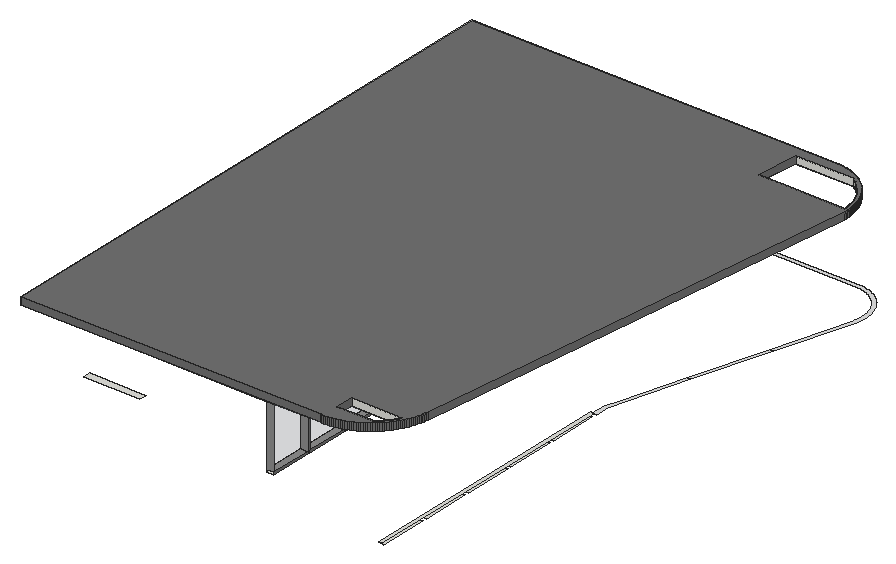
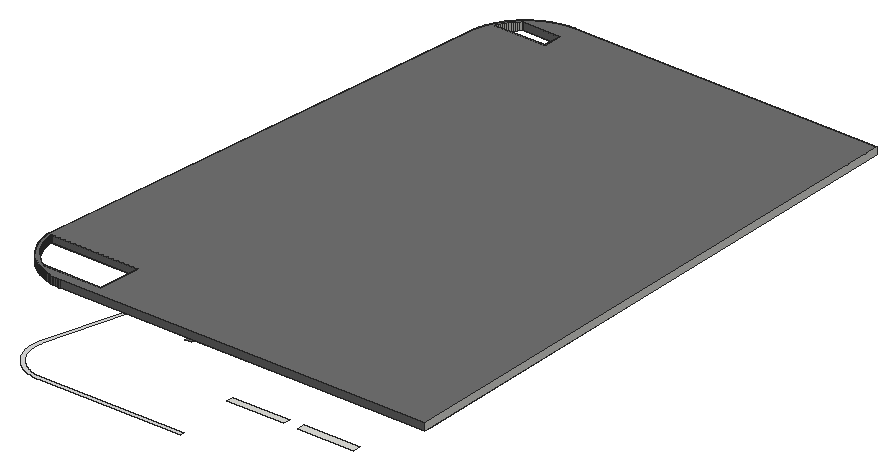
# SketchUp Ruby script. Lengths in inches.
U = 1.inch
M = Sketchup.active_model
def pt(a) = Geom::Point3d.new(a.map { |v| v * U })
def face(e, loops, mat)
  f = e.add_face(loops[0].map { |a| pt(a) })
  loops[1..].each { |l| e.add_face(l.map { |a| pt(a) }).erase! }
  f.material = f.back_material = mat if mat
  f
end
# faces: each face lists its corners as indices into pts; further lists are holes
def faces(e, pts, list, mat = nil) = list.each { |f| face(e, (f[0].is_a?(Array) ? f : [f]).map { |l| l.map { |i| pts[i] } }, mat) }
# xy, xz, yz: faces in a plane at the given z, y or x. An outline is a flat list of corners, or four numbers for a rectangle; further outlines are holes
def ring(l) = l.size == 4 ? [[l[0], l[1]], [l[2], l[1]], [l[2], l[3]], [l[0], l[3]]] : l.each_slice(2).to_a
def flat(e, list, mat, &to3) = list.each { |f| face(e, (f[0].is_a?(Array) ? f : [f]).map { |l| ring(l).map { |u, v| to3.(u, v) } }, mat) }
def xy(e, z, list, mat = nil) = flat(e, list, mat) { |x, y| [x, y, z] }
def xz(e, y, list, mat = nil) = flat(e, list, mat) { |x, z| [x, y, z] }
def yz(e, x, list, mat = nil) = flat(e, list, mat) { |y, z| [x, y, z] }
def lines(e, pts, list) = list.each { |a, b| e.add_line(pt(pts[a]), pt(pts[b])) }
# prism: a flat outline (further loops are holes) pulled along v
def prism(e, loops, v, mat = nil)
  f = face(e, loops, mat); d = Geom::Vector3d.new(v.map { |x| x * U })
  f.pushpull(f.normal.samedirection?(d) ? d.length : -d.length)
end
def box(e, o, s, mat = nil) = prism(e, [[o, [o[0] + s[0], o[1], o[2]], [o[0] + s[0], o[1] + s[1], o[2]], [o[0], o[1] + s[1], o[2]]]], [0, 0, s[2]], mat)
def at(x, y, z, deg = 0) = Geom::Transformation.translation(pt([x, y, z])) * Geom::Transformation.rotation(ORIGIN, Z_AXIS, deg.degrees)
def axes(o, x, y, z) = Geom::Transformation.new([*x, 0, *y, 0, *z, 0, *pt(o).to_a, 1])
def part(name) = M.definitions.add(name)
# library, detail: a bought-in or finely detailed component or shape, given as its bounding box
def library(name, o, s) = part(name).tap { |d| box(d.entities, o, s) }
def detail(e, o, s) = box(e.add_group.entities, o, s)
def put(e, d, t, mat = nil) = e.add_instance(d, t).tap { |i| i.material = mat if mat }
def group(e, t, mat = nil) = e.add_group.tap { |g| g.transformation = t; g.material = mat if mat }.entities
root = M.entities
M.materials.add("Glass_Basic_01").color = [105, 113, 122]
M.materials["Glass_Basic_01"].alpha = 0.25
M.materials.add("M01_Silver_Fog").color = [224, 224, 224]
M.materials.add("M04_Stone_Frost").color = [142, 142, 142]
M.materials.add("M06_Steel_Smoke").color = [114, 114, 114]
xy(root,682,[[300,8,303,49],[300,53,303,94],[300,98,303,139],[300,143,303,184],[300,188,303,229]])
xy(root,684,[[300,6,303,231]])
xy(root,684,[[302.38,231,305.51,231,305.51,243,324.34,307.35,321.22,307.35,306,255.36,303.26,246,302.38,243],[321.22,307.35,324.34,307.35,343.2,371.78,340.07,371.78],[340.07,371.78,343.2,371.78,362.06,436.22,362.32,437.22,362.58,438.42,362.79,439.63,362.96,440.85,363.08,442.08,363.16,443.31,363.1875,444.54,363.17,445.77,363.1,447,362.99,448.22,362.83,449.44,362.63,450.66,362.38,451.86,362.08,453.06,361.74,454.24,361.35,455.41,360.92,456.5625,360.45,457.7,359.93,458.82,359.37,459.91,358.77,460.99,358.13,462.03,358.13,462.04,357.45,463.0625,356.73,464.0625,355.97,465.03,355.18,465.98,355.17,465.98,354.35,466.89,353.49,467.76,352.59,468.61,351.67,469.42,350.71,470.19,349.72,470.93,348.71,471.63,347.67,472.29,346.61,472.91,345.52,473.49,344.41,474.03,343.29,474.52,342.14,474.97,340.98,475.38,339.8,475.75,338.61,476.0625,337.41,476.34,336.2,476.5625,334.99,476.74,333.76,476.88,332.53,476.97,331.5,477,210,477,210,474,331.45,474,332.38,473.97,333.49,473.89,334.6,473.77,335.71,473.6,336.8,473.4,337.89,473.15,338.97,472.86,340.04,472.53,341.09,472.16,342.13,471.75,343.16,471.3,344.16,470.82,345.15,470.29,346.11,469.73,347.05,469.13,347.97,468.5,348.87,467.83,349.74,467.125,350.58,466.39,351.39,465.62,352.17,464.83,352.92,464,353.64,463.14,354.33,462.26,354.98,461.36,355.6,460.43,356.18,459.47,356.73,458.5,357.23,457.5,357.7,456.49,358.13,455.46,358.52,454.41,358.875,453.35,359.18,452.28,359.45,451.2,359.68,450.1,359.87,449,360.01,447.89,360.11,446.78,360.17,445.67,360.1875,444.55,360.16,443.43,360.09,442.32,359.98,441.21,359.83,440.1,359.63,439,359.4,437.91,359.17,437.01]],"M01_Silver_Fog")
xy(root,703,[[204,7,210,43],[204,45,210,81],[204,83,210,119],[204,121,210,157],[204,159,210,195],
  [204,197,210,233]])
xy(root,705,[[204,7,210,43],[204,45,210,81],[204,83,210,119],[204,121,210,157],[204,159,210,195],
  [204,197,210,233]],"M04_Stone_Frost")
xy(root,725.98,[[54,0,102,6]])
xy(root,726,[[60,474,108,480],[120,474,168,480]])
xy(root,755,[[204,295,210,353],[204,355,210,413],[204,415,210,473]],"M06_Steel_Smoke")
xy(root,761,[[204,7,210,43],[204,45,210,81],[204,83,210,119],[204,121,210,157],[204,159,210,195],
  [204,197,210,233]])
xy(root,762,[[0,0,6,6],[6,0,204,6],[0,6,6,474],[6,6,12,474],[12,6,204,474],
  [204,234,210,240],[204,240,210,474],[0,474,6,480],[6,474,204,480],[204,474,210,480]])
xy(root,762,[[325.27,304.17,325.44,304.17,325.53,304.1875,325.62,304.2,325.7,304.22,325.79,304.25,325.87,304.28,326.03,304.36,326.24,304.51,326.3,304.57,326.42,304.71,326.52,304.85,326.5625,304.93,326.6,305.01,326.66,305.17,326.68,305.26,326.7,305.34,326.72,305.52,326.72,305.61,326.71,305.69,326.7,305.78,326.6875,305.87,326.67,305.95,326.64,306.04,326.61,306.12,326.53,306.28,326.43,306.42,326.375,306.49,326.31,306.55,326.25,306.61,326.18,306.67,326.04,306.77,325.96,306.8125,325.88,306.85,325.72,306.91,325.63,306.93,325.55,306.95,325.37,306.97,325.28,306.97,325.2,306.96,325.11,306.95,325.02,306.9375,324.9375,306.92,324.85,306.89,324.77,306.86,324.61,306.78,324.47,306.68,324.4,306.625,324.33,306.56,324.27,306.5,324.12,306.29,324,306.05,323.98,305.97,323.96,305.88,323.9375,305.8,323.93,305.71,323.92,305.62,323.92,305.53,323.93,305.44,323.9375,305.36,323.95,305.27,323.97,305.1875,324,305.1,324.03,305.02,324.11,304.86,324.26,304.65,324.32,304.58,324.39,304.52,324.6,304.37,324.84,304.25,324.92,304.23,325.01,304.2,325.09,304.1875,325.18,304.18],[326.2,307.35,326.375,307.35,326.46,307.36,326.55,307.38,326.63,307.4,326.72,307.43,326.8,307.46,326.96,307.54,327.17,307.69,327.3,307.82,327.35,307.88,327.4,307.96,327.45,308.03,327.49,308.11,327.53,308.1875,327.56,308.27,327.59,308.35,327.61,308.4375,327.63,308.52,327.65,308.7,327.65,308.79,327.63,308.96,327.62,309.05,327.6,309.13,327.57,309.22,327.54,309.3,327.46,309.46,327.31,309.67,327.25,309.73,327.11,309.85,326.97,309.95,326.89,309.99,326.8125,310.03,326.73,310.0625,326.65,310.09,326.5625,310.11,326.48,310.13,326.3,310.15,326.21,310.15,326.04,310.13,325.95,310.12,325.87,310.1,325.78,310.07,325.7,310.04,325.54,309.96,325.4,309.86,325.33,309.8,325.27,309.74,325.2,309.68,325.05,309.47,325.01,309.39,324.97,309.3125,324.9375,309.23,324.91,309.15,324.89,309.0625,324.87,308.98,324.85,308.8,324.85,308.71,324.87,308.54,324.88,308.45,324.9,308.37,324.93,308.28,324.96,308.2,325.04,308.04,325.14,307.9,325.26,307.76,325.32,307.7,325.53,307.55,325.61,307.5,325.6875,307.47,325.77,307.43,325.85,307.41,325.9375,307.38,326.02,307.37]],"M01_Silver_Fog")
xy(root,762,[[[204,0,204,234,210,234,210,480,309.87,480,311.01,479.97,312.52,479.88,314.03,479.75,315.54,479.56,317.04,479.33,318.53,479.04,320.01,478.71,321.48,478.33,322.9375,477.91,324.38,477.43,325.8,476.92,327.21,476.35,328.6,475.74,329.97,475.09,331.32,474.39,332.01,474,332.64,473.65,333.94,472.86,335.21,472.04,336.46,471.17,337.68,470.26,338.86,469.32,340.02,468.34,341.14,467.32,342.23,466.26,343.29,465.17,344.31,464.05,345.29,462.89,346.24,461.7,347.14,460.49,348.01,459.24,348.84,457.97,349.62,456.67,350.36,455.34,351.06,454,351.71,452.63,352.32,451.24,352.89,449.83,353.41,448.41,353.88,446.96,354.31,445.51,354.68,444.04,355.02,442.56,355.3,441.07,355.53,439.57,355.72,438.06,355.86,436.55,355.94,435.03,355.97,433.9,355.97,432,308.97,47.65,308.77,46.08,308.52,44.53,308.42,44,308.23,42.98,307.89,41.45,307.5,39.92,307.08,38.4,306.6,36.9,306.09,35.42,305.53,33.94,305.23,33.22,304.92,32.49,304.28,31.05,303.59,29.64,302.86,28.24,302.1,26.87,301.29,25.52,300.44,24.1875,299.56,22.89,298.63,21.61,297.67,20.37,296.67,19.15,295.64,17.96,294.58,16.8,293.48,15.67,292.35,14.58,291.18,13.52,289.99,12.49,289.5,12.1,288.77,11.5,287.51,10.55,286.23,9.63,284.93,8.75,283.6,7.91,282.24,7.11,280.87,6.34,280.2,6,279.47,5.625,278.05,4.94,276.61,4.31,275.15,3.71,273.68,3.16,272.1875,2.65,270.68,2.18,269.17,1.76,267.64,1.38,266.1,1.05,264.55,0.76,263,0.52,261.43,0.33,259.87,0.18,258.3,0.07,256.72,0.01,255.15,0],[352.9375,435.02,352.86,436.33,352.74,437.74,352.5625,439.15,352.34,440.55,352.08,441.95,351.77,443.34,351.41,444.71,351.01,446.07,350.57,447.42,350.09,448.76,349.56,450.08,348.99,451.38,348.375,452.66,347.72,453.92,347.03,455.16,346.29,456.375,345.52,457.57,344.71,458.73,343.86,459.875,342.98,460.98,342.06,462.07,341.1,463.12,340.11,464.14,339.09,465.13,338.04,466.08,336.96,467,335.85,467.89,334.71,468.73,333.54,469.55,332.35,470.32,331.22,471,282.97,471,279.34,435.58],[257.49,15.1,288.42,15.1,289.19,15.76,290.29,16.77,291.36,17.8,292.4,18.86,293.41,19.96,294.38,21.08,295.32,22.23,296.23,23.41,297.1,24.61,297.9375,25.84,298.74,27.09,299.5,28.37,300.22,29.67,300.51,30.22,257.49,30.22],[325.27,304.17,325.44,304.17,325.53,304.1875,325.62,304.2,325.7,304.22,325.79,304.25,325.87,304.28,326.03,304.36,326.24,304.51,326.3,304.57,326.42,304.71,326.52,304.85,326.5625,304.93,326.6,305.01,326.66,305.17,326.68,305.26,326.7,305.34,326.72,305.52,326.72,305.61,326.71,305.69,326.7,305.78,326.6875,305.87,326.67,305.95,326.64,306.04,326.61,306.12,326.53,306.28,326.43,306.42,326.375,306.49,326.31,306.55,326.25,306.61,326.18,306.67,326.04,306.77,325.96,306.8125,325.88,306.85,325.72,306.91,325.63,306.93,325.55,306.95,325.37,306.97,325.28,306.97,325.2,306.96,325.11,306.95,325.02,306.9375,324.9375,306.92,324.85,306.89,324.77,306.86,324.61,306.78,324.47,306.68,324.4,306.625,324.33,306.56,324.27,306.5,324.12,306.29,324,306.05,323.98,305.97,323.96,305.88,323.9375,305.8,323.93,305.71,323.92,305.62,323.92,305.53,323.93,305.44,323.9375,305.36,323.95,305.27,323.97,305.1875,324,305.1,324.03,305.02,324.11,304.86,324.26,304.65,324.32,304.58,324.39,304.52,324.6,304.37,324.84,304.25,324.92,304.23,325.01,304.2,325.09,304.1875,325.18,304.18],[326.2,307.35,326.375,307.35,326.46,307.36,326.55,307.38,326.63,307.4,326.72,307.43,326.8,307.46,326.96,307.54,327.17,307.69,327.3,307.82,327.35,307.88,327.4,307.96,327.45,308.03,327.49,308.11,327.53,308.1875,327.56,308.27,327.59,308.35,327.61,308.4375,327.63,308.52,327.65,308.7,327.65,308.79,327.63,308.96,327.62,309.05,327.6,309.13,327.57,309.22,327.54,309.3,327.46,309.46,327.31,309.67,327.25,309.73,327.11,309.85,326.97,309.95,326.89,309.99,326.8125,310.03,326.73,310.0625,326.65,310.09,326.5625,310.11,326.48,310.13,326.3,310.15,326.21,310.15,326.04,310.13,325.95,310.12,325.87,310.1,325.78,310.07,325.7,310.04,325.54,309.96,325.4,309.86,325.33,309.8,325.27,309.74,325.2,309.68,325.05,309.47,325.01,309.39,324.97,309.3125,324.9375,309.23,324.91,309.15,324.89,309.0625,324.87,308.98,324.85,308.8,324.85,308.71,324.87,308.54,324.88,308.45,324.9,308.37,324.93,308.28,324.96,308.2,325.04,308.04,325.14,307.9,325.26,307.76,325.32,307.7,325.53,307.55,325.61,307.5,325.6875,307.47,325.77,307.43,325.85,307.41,325.9375,307.38,326.02,307.37]]],"M06_Steel_Smoke")
xy(root,768,[[[0,0,255.15,0,256.72,0.01,258.3,0.07,259.87,0.18,261.43,0.33,263,0.52,264.55,0.76,266.1,1.05,267.64,1.38,269.17,1.76,270.68,2.18,272.1875,2.65,273.68,3.16,275.15,3.71,276.61,4.31,278.05,4.94,279.47,5.625,280.87,6.34,282.24,7.11,283.6,7.91,284.93,8.75,286.23,9.63,287.51,10.55,288.77,11.5,289.99,12.49,291.18,13.52,292.35,14.58,293.48,15.67,294.58,16.8,295.64,17.96,296.67,19.15,297.67,20.37,298.63,21.61,299.56,22.89,300.44,24.1875,301.29,25.52,302.1,26.87,302.86,28.24,303.59,29.64,304.28,31.05,304.92,32.49,305.53,33.94,306.09,35.42,306.6,36.9,307.08,38.4,307.5,39.92,307.89,41.45,308.23,42.98,308.52,44.53,308.77,46.08,308.97,47.65,355.97,432,355.97,433.9,355.94,435.03,355.86,436.55,355.72,438.06,355.53,439.57,355.3,441.07,355.02,442.56,354.68,444.04,354.31,445.51,353.88,446.96,353.41,448.41,352.89,449.83,352.32,451.24,351.71,452.63,351.06,454,350.36,455.34,349.62,456.67,348.84,457.97,348.01,459.24,347.14,460.49,346.24,461.7,345.29,462.89,344.31,464.05,343.29,465.17,342.23,466.26,341.14,467.32,340.02,468.34,338.86,469.32,337.68,470.26,336.46,471.17,335.21,472.04,333.94,472.86,332.64,473.65,331.32,474.39,329.97,475.09,328.6,475.74,327.21,476.35,325.8,476.92,324.38,477.43,322.9375,477.91,321.48,478.33,320.01,478.71,318.53,479.04,317.04,479.33,315.54,479.56,314.03,479.75,312.52,479.88,311.01,479.97,309.87,480,0,480],[352.9375,435.02,279.34,435.58,282.97,471,331.22,471,332.35,470.32,333.54,469.55,334.71,468.73,335.85,467.89,336.96,467,338.04,466.08,339.09,465.13,340.11,464.14,341.1,463.12,342.06,462.07,342.98,460.98,343.86,459.875,344.71,458.73,345.52,457.57,346.29,456.375,347.03,455.16,347.72,453.92,348.375,452.66,348.99,451.38,349.56,450.08,350.09,448.76,350.57,447.42,351.01,446.07,351.41,444.71,351.77,443.34,352.08,441.95,352.34,440.55,352.5625,439.15,352.74,437.74,352.86,436.33],[257.49,15.1,257.49,30.22,300.51,30.22,300.22,29.67,299.5,28.37,298.74,27.09,297.9375,25.84,297.1,24.61,296.23,23.41,295.32,22.23,294.38,21.08,293.41,19.96,292.4,18.86,291.36,17.8,290.29,16.77,289.19,15.76,288.42,15.1]]],"M06_Steel_Smoke")
xz(root,0,[[0,762,255.15,768]],"M06_Steel_Smoke")
xz(root,7,[[204,705,210,761]],"M04_Stone_Frost")
xz(root,15.1,[[257.49,762,288.42,768]],"M06_Steel_Smoke")
xz(root,30.22,[[257.49,762,300.51,768]])
xz(root,43,[[204,705,210,761]],"M04_Stone_Frost")
xz(root,45,[[204,705,210,761]],"M04_Stone_Frost")
xz(root,81,[[204,705,210,761]],"M04_Stone_Frost")
xz(root,83,[[204,705,210,761]],"M04_Stone_Frost")
xz(root,119,[[204,705,210,761]],"M04_Stone_Frost")
xz(root,121,[[204,705,210,761]],"M04_Stone_Frost")
xz(root,157,[[204,705,210,761]],"M04_Stone_Frost")
xz(root,159,[[204,705,210,761]],"M04_Stone_Frost")
xz(root,195,[[204,705,210,761]],"M04_Stone_Frost")
xz(root,197,[[204,705,210,761]],"M04_Stone_Frost")
xz(root,233,[[204,705,210,761]],"M04_Stone_Frost")
xz(root,471,[[282.97,762,331.22,768]])
xz(root,480,[[0,762,309.87,768]],"M06_Steel_Smoke")
yz(root,0,[[0,762,480,768]])
yz(root,204,[[7,705,43,761],[45,705,81,761],[83,705,119,761],[121,705,157,761],[159,705,195,761],
  [197,705,233,761]],"Glass_Basic_01")
yz(root,210,[[7,703,43,705],[45,703,81,705],[83,703,119,705],[121,703,157,705],[159,703,195,705],
  [197,703,231,705],[44,705,45,705,45,761,81,761,81,705,82,705,82,762,44,762],[82,705,83,705,83,761,119,761,119,705,120,705,120,762,82,762],[120,705,121,705,121,761,157,761,157,705,158,705,158,762,120,762],[158,705,159,705,159,761,195,761,195,705,196,705,196,762,158,762],
  [196,705,197,705,197,761,231,761,231,762,196,762],[231,705,233,761]],"M06_Steel_Smoke")
yz(root,257.49,[[15.1,762,30.22,768]],"M06_Steel_Smoke")
yz(root,355.97,[[432,762,433.9,768]],"M06_Steel_Smoke")
p = [[256.72,0.01,768],[255.15,0,768],[255.15,0,762],[256.72,0.01,762],[258.3,0.07,768],[258.3,0.07,762],
  [259.87,0.18,768],[259.87,0.18,762],[261.43,0.33,768],[261.43,0.33,762],[263,0.52,768],[263,0.52,762],
  [264.55,0.76,768],[264.55,0.76,762],[266.1,1.05,768],[266.1,1.05,762],[267.64,1.38,768],[267.64,1.38,762],
  [269.17,1.76,768],[269.17,1.76,762],[270.68,2.18,768],[270.68,2.18,762],[272.1875,2.65,768],[272.1875,2.65,762],
  [273.68,3.16,768],[273.68,3.16,762],[275.15,3.71,768],[275.15,3.71,762],[276.61,4.31,768],[276.61,4.31,762],
  [278.05,4.94,768],[278.05,4.94,762],[279.47,5.625,768],[279.47,5.625,762],[280.87,6.34,768],[280.2,6,762],
  [280.87,6.34,762],[282.24,7.11,768],[282.24,7.11,762],[283.6,7.91,768],[283.6,7.91,762],[284.93,8.75,768],
  [284.93,8.75,762],[286.23,9.63,768],[286.23,9.63,762],[287.51,10.55,768],[287.51,10.55,762],[288.77,11.5,768],
  [288.77,11.5,762],[289.99,12.49,768],[289.5,12.1,762],[289.99,12.49,762],[291.18,13.52,768],[291.18,13.52,762],
  [292.35,14.58,768],[292.35,14.58,762],[293.48,15.67,768],[293.48,15.67,762],[289.19,15.76,762],[288.42,15.1,762],
  [288.42,15.1,768],[289.19,15.76,768],[294.58,16.8,768],[294.58,16.8,762],[290.29,16.77,762],[290.29,16.77,768],
  [291.36,17.8,762],[291.36,17.8,768],[295.64,17.96,768],[295.64,17.96,762],[292.4,18.86,762],[292.4,18.86,768],
  [296.67,19.15,768],[296.67,19.15,762],[293.41,19.96,762],[293.41,19.96,768],[297.67,20.37,768],[297.67,20.37,762],
  [294.38,21.08,762],[294.38,21.08,768],[298.63,21.61,768],[298.63,21.61,762],[295.32,22.23,762],[295.32,22.23,768],
  [299.56,22.89,768],[299.56,22.89,762],[296.23,23.41,762],[296.23,23.41,768],[300.44,24.1875,768],[300.44,24.1875,762],
  [297.1,24.61,762],[297.1,24.61,768],[301.29,25.52,768],[301.29,25.52,762],[297.9375,25.84,762],[297.9375,25.84,768],
  [302.1,26.87,768],[302.1,26.87,762],[298.74,27.09,762],[298.74,27.09,768],[302.86,28.24,768],[302.86,28.24,762],
  [299.5,28.37,762],[299.5,28.37,768],[303.59,29.64,768],[303.59,29.64,762],[300.22,29.67,762],[300.22,29.67,768],
  [304.28,31.05,768],[304.28,31.05,762],[300.51,30.22,762],[300.51,30.22,768],[304.92,32.49,768],[304.92,32.49,762],
  [305.53,33.94,768],[305.23,33.22,762],[305.53,33.94,762],[306.09,35.42,768],[306.09,35.42,762],[306.6,36.9,768],
  [306.6,36.9,762],[307.08,38.4,768],[307.08,38.4,762],[307.5,39.92,768],[307.5,39.92,762],[307.89,41.45,768],
  [307.89,41.45,762],[308.23,42.98,768],[308.23,42.98,762],[308.52,44.53,768],[308.42,44,762],[308.52,44.53,762],
  [308.77,46.08,768],[308.77,46.08,762],[308.97,47.65,768],[308.97,47.65,762],[355.97,432,762],[355.97,432,768],
  [355.94,435.03,768],[355.97,433.9,768],[355.97,433.9,762],[355.94,435.03,762],[352.9375,435.02,762],[279.34,435.58,762],
  [279.34,435.58,768],[352.9375,435.02,768],[352.86,436.33,762],[352.86,436.33,768],[355.86,436.55,768],[355.86,436.55,762],
  [282.97,471,762],[282.97,471,768],[352.74,437.74,762],[352.74,437.74,768],[355.72,438.06,768],[355.72,438.06,762],
  [352.5625,439.15,762],[352.5625,439.15,768],[355.53,439.57,768],[355.53,439.57,762],[352.34,440.55,762],[352.34,440.55,768],
  [355.3,441.07,768],[355.3,441.07,762],[352.08,441.95,762],[352.08,441.95,768],[355.02,442.56,768],[355.02,442.56,762],
  [351.77,443.34,762],[351.77,443.34,768],[354.68,444.04,768],[354.68,444.04,762],[351.41,444.71,762],[351.41,444.71,768],
  [354.31,445.51,768],[354.31,445.51,762],[351.01,446.07,762],[351.01,446.07,768],[353.88,446.96,768],[353.88,446.96,762],
  [350.57,447.42,762],[350.57,447.42,768],[353.41,448.41,768],[353.41,448.41,762],[350.09,448.76,762],[350.09,448.76,768],
  [352.89,449.83,768],[352.89,449.83,762],[349.56,450.08,762],[349.56,450.08,768],[352.32,451.24,768],[352.32,451.24,762],
  [348.99,451.38,762],[348.99,451.38,768],[351.71,452.63,768],[351.71,452.63,762],[348.375,452.66,762],[348.375,452.66,768],
  [351.06,454,768],[351.06,454,762],[347.72,453.92,762],[347.72,453.92,768],[347.03,455.16,762],[347.03,455.16,768],
  [350.36,455.34,768],[350.36,455.34,762],[346.29,456.375,762],[346.29,456.375,768],[349.62,456.67,768],[349.62,456.67,762],
  [345.52,457.57,762],[345.52,457.57,768],[348.84,457.97,768],[348.84,457.97,762],[344.71,458.73,762],[344.71,458.73,768],
  [348.01,459.24,768],[348.01,459.24,762],[343.86,459.875,762],[343.86,459.875,768],[347.14,460.49,768],[347.14,460.49,762],
  [342.98,460.98,762],[342.98,460.98,768],[346.24,461.7,768],[346.24,461.7,762],[342.06,462.07,762],[342.06,462.07,768],
  [345.29,462.89,768],[345.29,462.89,762],[341.1,463.12,762],[341.1,463.12,768],[344.31,464.05,768],[344.31,464.05,762],
  [340.11,464.14,762],[340.11,464.14,768],[343.29,465.17,768],[343.29,465.17,762],[339.09,465.13,762],[339.09,465.13,768],
  [338.04,466.08,762],[338.04,466.08,768],[342.23,466.26,768],[342.23,466.26,762],[336.96,467,762],[336.96,467,768],
  [341.14,467.32,768],[341.14,467.32,762],[335.85,467.89,762],[335.85,467.89,768],[340.02,468.34,768],[340.02,468.34,762],
  [334.71,468.73,762],[334.71,468.73,768],[338.86,469.32,768],[338.86,469.32,762],[333.54,469.55,762],[333.54,469.55,768],
  [337.68,470.26,768],[337.68,470.26,762],[332.35,470.32,762],[332.35,470.32,768],[331.22,471,762],[331.22,471,768],
  [336.46,471.17,768],[336.46,471.17,762],[335.21,472.04,768],[335.21,472.04,762],[333.94,472.86,768],[333.94,472.86,762],
  [332.64,473.65,768],[332.64,473.65,762],[331.32,474.39,768],[332.01,474,762],[331.32,474.39,762],[329.97,475.09,768],
  [329.97,475.09,762],[328.6,475.74,768],[328.6,475.74,762],[327.21,476.35,768],[327.21,476.35,762],[325.8,476.92,768],
  [325.8,476.92,762],[324.38,477.43,768],[324.38,477.43,762],[322.9375,477.91,768],[322.9375,477.91,762],[321.48,478.33,768],
  [321.48,478.33,762],[320.01,478.71,768],[320.01,478.71,762],[318.53,479.04,768],[318.53,479.04,762],[317.04,479.33,768],
  [317.04,479.33,762],[315.54,479.56,768],[315.54,479.56,762],[314.03,479.75,768],[314.03,479.75,762],[312.52,479.88,768],
  [312.52,479.88,762],[311.01,479.97,768],[311.01,479.97,762],[309.87,480,768],[309.87,480,762],[308.53,44,762],
  [289.59,12.1,762],[305.53,33.22,762]]
faces(root,p,[[0,1,2,3],[4,0,3,5],[6,4,5,7],[8,6,7,9],[10,8,9,11],[12,10,11,13],[14,12,13,15],[16,14,15,17],
  [18,16,17,19],[20,18,19,21],[22,20,21,23],[24,22,23,25],[26,24,25,27],[28,26,27,29],[30,28,29,31],[32,30,31,33],
  [34,32,33,35,36],[37,34,36,38],[39,37,38,40],[41,39,40,42],[43,41,42,44],[45,43,44,46],[47,45,46,48],[49,47,48,50,51],
  [52,49,51,53],[54,52,53,55],[56,54,55,57],[62,56,57,63],[68,62,63,69],[72,68,69,73],[76,72,73,77],[80,76,77,81],
  [84,80,81,85],[88,84,85,89],[92,88,89,93],[96,92,93,97],[100,96,97,101],[104,100,101,105],[108,104,105,109],[112,108,109,113],
  [114,112,113,115,116],[117,114,116,118],[119,117,118,120],[121,119,120,122],[123,121,122,124],[125,123,124,126],[127,125,126,128],[129,127,128,130,131],
  [132,129,131,133],[134,132,133,135],[134,135,136,137],[138,139,140,141],[142,143,144,145],[148,138,141,149],[143,150,151,144],[154,148,149,155],
  [158,154,155,159],[162,158,159,163],[166,162,163,167],[170,166,167,171],[174,170,171,175],[178,174,175,179],[182,178,179,183],[186,182,183,187],
  [190,186,187,191],[194,190,191,195],[198,194,195,199],[204,198,199,205],[208,204,205,209],[212,208,209,213],[216,212,213,217],[220,216,217,221],
  [224,220,221,225],[228,224,225,229],[232,228,229,233],[236,232,233,237],[242,236,237,243],[246,242,243,247],[250,246,247,251],[254,250,251,255],
  [258,254,255,259],[264,258,259,265],[266,264,265,267],[268,266,267,269],[270,268,269,271],[272,270,271,273,274],[275,272,274,276],[277,275,276,278],
  [279,277,278,280],[281,279,280,282],[283,281,282,284],[285,283,284,286],[287,285,286,288],[289,287,288,290],[291,289,290,292],[293,291,292,294],
  [295,293,294,296],[297,295,296,298],[299,297,298,300],[301,299,300,302],[303,301,302,304]],"M06_Steel_Smoke")
faces(root,p,[[58,59,60,61],[64,58,61,65],[66,64,65,67],[70,66,67,71],[74,70,71,75],[78,74,75,79],[82,78,79,83],[86,82,83,87],
  [90,86,87,91],[94,90,91,95],[98,94,95,99],[102,98,99,103],[106,102,103,107],[110,106,107,111],[146,142,145,147],[152,146,147,153],
  [156,152,153,157],[160,156,157,161],[164,160,161,165],[168,164,165,169],[172,168,169,173],[176,172,173,177],[180,176,177,181],[184,180,181,185],
  [188,184,185,189],[192,188,189,193],[196,192,193,197],[200,196,197,201],[202,200,201,203],[206,202,203,207],[210,206,207,211],[214,210,211,215],
  [218,214,215,219],[222,218,219,223],[226,222,223,227],[230,226,227,231],[234,230,231,235],[238,234,235,239],[240,238,239,241],[244,240,241,245],
  [248,244,245,249],[252,248,249,253],[256,252,253,257],[260,256,257,261],[262,260,261,263]])
lines(root,p,[[130,305],[50,306],[115,307]])
